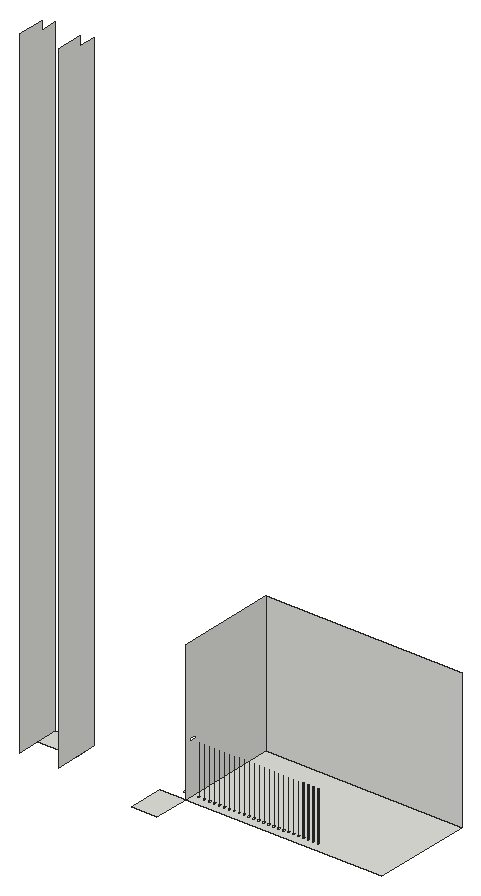
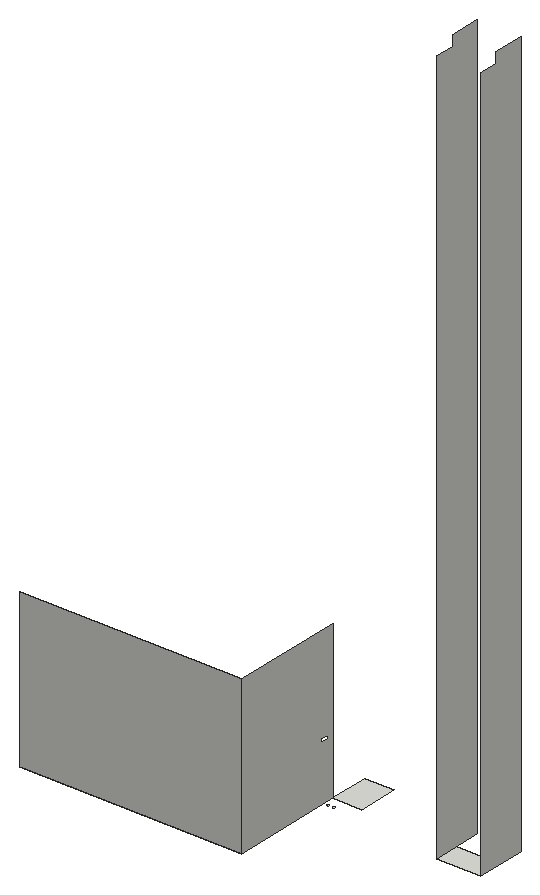
# SketchUp Ruby script. Lengths in inches.
U = 1.inch
M = Sketchup.active_model
def pt(a) = Geom::Point3d.new(a.map { |v| v * U })
def face(e, loops, mat)
  f = e.add_face(loops[0].map { |a| pt(a) })
  loops[1..].each { |l| e.add_face(l.map { |a| pt(a) }).erase! }
  f.material = f.back_material = mat if mat
  f
end
# faces: each face lists its corners as indices into pts; further lists are holes
def faces(e, pts, list, mat = nil) = list.each { |f| face(e, (f[0].is_a?(Array) ? f : [f]).map { |l| l.map { |i| pts[i] } }, mat) }
# xy, xz, yz: faces in a plane at the given z, y or x. An outline is a flat list of corners, or four numbers for a rectangle; further outlines are holes
def ring(l) = l.size == 4 ? [[l[0], l[1]], [l[2], l[1]], [l[2], l[3]], [l[0], l[3]]] : l.each_slice(2).to_a
def flat(e, list, mat, &to3) = list.each { |f| face(e, (f[0].is_a?(Array) ? f : [f]).map { |l| ring(l).map { |u, v| to3.(u, v) } }, mat) }
def xy(e, z, list, mat = nil) = flat(e, list, mat) { |x, y| [x, y, z] }
def xz(e, y, list, mat = nil) = flat(e, list, mat) { |x, z| [x, y, z] }
def yz(e, x, list, mat = nil) = flat(e, list, mat) { |y, z| [x, y, z] }
def lines(e, pts, list) = list.each { |a, b| e.add_line(pt(pts[a]), pt(pts[b])) }
# prism: a flat outline (further loops are holes) pulled along v
def prism(e, loops, v, mat = nil)
  f = face(e, loops, mat); d = Geom::Vector3d.new(v.map { |x| x * U })
  f.pushpull(f.normal.samedirection?(d) ? d.length : -d.length)
end
def box(e, o, s, mat = nil) = prism(e, [[o, [o[0] + s[0], o[1], o[2]], [o[0] + s[0], o[1] + s[1], o[2]], [o[0], o[1] + s[1], o[2]]]], [0, 0, s[2]], mat)
def at(x, y, z, deg = 0) = Geom::Transformation.translation(pt([x, y, z])) * Geom::Transformation.rotation(ORIGIN, Z_AXIS, deg.degrees)
def axes(o, x, y, z) = Geom::Transformation.new([*x, 0, *y, 0, *z, 0, *pt(o).to_a, 1])
def part(name) = M.definitions.add(name)
# library, detail: a bought-in or finely detailed component or shape, given as its bounding box
def library(name, o, s) = part(name).tap { |d| box(d.entities, o, s) }
def detail(e, o, s) = box(e.add_group.entities, o, s)
def put(e, d, t, mat = nil) = e.add_instance(d, t).tap { |i| i.material = mat if mat }
def group(e, t, mat = nil) = e.add_group.tap { |g| g.transformation = t; g.material = mat if mat }.entities
root = M.entities
xy(root,204.9375,[[259.3125,81.125,290.4375,124.5],[110.7,124.5,157.47,150.6875],[[290.4375,124.5,528.75,246],[520.27,135.31,520.48,135.34,520.67,135.42,520.84,135.55,520.97,135.72,521.05,135.91,521.08,136.12,521.05,136.33,520.97,136.53,520.84,136.7,520.67,136.83,520.48,136.91,520.27,136.93,520.06,136.91,519.86,136.83,519.69,136.7,519.5625,136.53,519.48,136.33,519.45,136.12,519.48,135.91,519.5625,135.72,519.69,135.55,519.86,135.42,520.06,135.34],[514.2,135.31,514.41,135.34,514.61,135.42,514.78,135.55,514.91,135.72,514.99,135.91,515.02,136.12,514.99,136.33,514.91,136.53,514.78,136.7,514.61,136.83,514.41,136.91,514.2,136.93,513.99,136.91,513.8,136.83,513.63,136.7,513.5,136.53,513.42,136.33,513.39,136.12,513.42,135.91,513.5,135.72,513.63,135.55,513.8,135.42,513.99,135.34],[508.14,135.31,508.35,135.34,508.55,135.42,508.72,135.55,508.85,135.72,508.93,135.91,508.95,136.12,508.93,136.33,508.85,136.53,508.72,136.7,508.55,136.83,508.35,136.91,508.14,136.93,507.93,136.91,507.74,136.83,507.57,136.7,507.4375,136.53,507.36,136.33,507.33,136.12,507.36,135.91,507.4375,135.72,507.57,135.55,507.74,135.42,507.93,135.34],[502.27,135.31,502.48,135.34,502.67,135.42,502.84,135.55,502.97,135.72,503.05,135.91,503.08,136.12,503.05,136.33,502.97,136.53,502.84,136.7,502.67,136.83,502.48,136.91,502.27,136.93,502.06,136.91,501.86,136.83,501.69,136.7,501.5625,136.53,501.48,136.33,501.45,136.12,501.48,135.91,501.5625,135.72,501.69,135.55,501.86,135.42,502.06,135.34],[496.27,135.31,496.48,135.34,496.67,135.42,496.84,135.55,496.97,135.72,497.05,135.91,497.08,136.12,497.05,136.33,496.97,136.53,496.84,136.7,496.67,136.83,496.48,136.91,496.27,136.93,496.06,136.91,495.86,136.83,495.69,136.7,495.5625,136.53,495.48,136.33,495.45,136.12,495.48,135.91,495.5625,135.72,495.69,135.55,495.86,135.42,496.06,135.34],[490.27,135.31,490.48,135.34,490.67,135.42,490.84,135.55,490.97,135.72,491.05,135.91,491.08,136.12,491.05,136.33,490.97,136.53,490.84,136.7,490.67,136.83,490.48,136.91,490.27,136.93,490.06,136.91,489.86,136.83,489.69,136.7,489.5625,136.53,489.48,136.33,489.45,136.12,489.48,135.91,489.5625,135.72,489.69,135.55,489.86,135.42,490.06,135.34],[484.2,135.31,484.41,135.34,484.61,135.42,484.78,135.55,484.91,135.72,484.99,135.91,485.02,136.12,484.99,136.33,484.91,136.53,484.78,136.7,484.61,136.83,484.41,136.91,484.2,136.93,483.99,136.91,483.8,136.83,483.63,136.7,483.5,136.53,483.42,136.33,483.39,136.12,483.42,135.91,483.5,135.72,483.63,135.55,483.8,135.42,483.99,135.34],[478.27,135.31,478.48,135.34,478.67,135.42,478.84,135.55,478.97,135.72,479.05,135.91,479.08,136.12,479.05,136.33,478.97,136.53,478.84,136.7,478.67,136.83,478.48,136.91,478.27,136.93,478.06,136.91,477.86,136.83,477.69,136.7,477.5625,136.53,477.48,136.33,477.45,136.12,477.48,135.91,477.5625,135.72,477.69,135.55,477.86,135.42,478.06,135.34],[472.27,135.31,472.48,135.34,472.67,135.42,472.84,135.55,472.97,135.72,473.05,135.91,473.08,136.12,473.05,136.33,472.97,136.53,472.84,136.7,472.67,136.83,472.48,136.91,472.27,136.93,472.06,136.91,471.86,136.83,471.69,136.7,471.5625,136.53,471.48,136.33,471.45,136.12,471.48,135.91,471.5625,135.72,471.69,135.55,471.86,135.42,472.06,135.34],[466.27,135.31,466.48,135.34,466.67,135.42,466.84,135.55,466.97,135.72,467.05,135.91,467.08,136.12,467.05,136.33,466.97,136.53,466.84,136.7,466.67,136.83,466.48,136.91,466.27,136.93,466.06,136.91,465.86,136.83,465.69,136.7,465.5625,136.53,465.48,136.33,465.45,136.12,465.48,135.91,465.5625,135.72,465.69,135.55,465.86,135.42,466.06,135.34],[460.33,135.31,460.54,135.34,460.74,135.42,460.9,135.55,461.03,135.72,461.11,135.91,461.14,136.12,461.11,136.33,461.03,136.53,460.9,136.7,460.74,136.83,460.54,136.91,460.33,136.93,460.12,136.91,459.92,136.83,459.75,136.7,459.625,136.53,459.54,136.33,459.52,136.12,459.54,135.91,459.625,135.72,459.75,135.55,459.92,135.42,460.12,135.34],[454.33,135.31,454.54,135.34,454.74,135.42,454.9,135.55,455.03,135.72,455.11,135.91,455.14,136.12,455.11,136.33,455.03,136.53,454.9,136.7,454.74,136.83,454.54,136.91,454.33,136.93,454.12,136.91,453.92,136.83,453.75,136.7,453.625,136.53,453.54,136.33,453.52,136.12,453.54,135.91,453.625,135.72,453.75,135.55,453.92,135.42,454.12,135.34],[448.33,135.31,448.54,135.34,448.74,135.42,448.9,135.55,449.03,135.72,449.11,135.91,449.14,136.12,449.11,136.33,449.03,136.53,448.9,136.7,448.74,136.83,448.54,136.91,448.33,136.93,448.12,136.91,447.92,136.83,447.75,136.7,447.625,136.53,447.54,136.33,447.52,136.12,447.54,135.91,447.625,135.72,447.75,135.55,447.92,135.42,448.12,135.34],[442.33,135.31,442.54,135.34,442.74,135.42,442.9,135.55,443.03,135.72,443.11,135.91,443.14,136.12,443.11,136.33,443.03,136.53,442.9,136.7,442.74,136.83,442.54,136.91,442.33,136.93,442.12,136.91,441.92,136.83,441.75,136.7,441.625,136.53,441.54,136.33,441.52,136.12,441.54,135.91,441.625,135.72,441.75,135.55,441.92,135.42,442.12,135.34],[436.33,135.31,436.54,135.34,436.74,135.42,436.9,135.55,437.03,135.72,437.11,135.91,437.14,136.12,437.11,136.33,437.03,136.53,436.9,136.7,436.74,136.83,436.54,136.91,436.33,136.93,436.12,136.91,435.92,136.83,435.75,136.7,435.625,136.53,435.54,136.33,435.52,136.12,435.54,135.91,435.625,135.72,435.75,135.55,435.92,135.42,436.12,135.34],[430.33,135.31,430.54,135.34,430.74,135.42,430.9,135.55,431.03,135.72,431.11,135.91,431.14,136.12,431.11,136.33,431.03,136.53,430.9,136.7,430.74,136.83,430.54,136.91,430.33,136.93,430.12,136.91,429.92,136.83,429.75,136.7,429.625,136.53,429.54,136.33,429.52,136.12,429.54,135.91,429.625,135.72,429.75,135.55,429.92,135.42,430.12,135.34],[424.33,135.31,424.54,135.34,424.74,135.42,424.9,135.55,425.03,135.72,425.11,135.91,425.14,136.12,425.11,136.33,425.03,136.53,424.9,136.7,424.74,136.83,424.54,136.91,424.33,136.93,424.12,136.91,423.92,136.83,423.75,136.7,423.625,136.53,423.54,136.33,423.52,136.12,423.54,135.91,423.625,135.72,423.75,135.55,423.92,135.42,424.12,135.34],[418.33,135.31,418.54,135.34,418.74,135.42,418.9,135.55,419.03,135.72,419.11,135.91,419.14,136.12,419.11,136.33,419.03,136.53,418.9,136.7,418.74,136.83,418.54,136.91,418.33,136.93,418.12,136.91,417.92,136.83,417.75,136.7,417.625,136.53,417.54,136.33,417.52,136.12,417.54,135.91,417.625,135.72,417.75,135.55,417.92,135.42,418.12,135.34],[412.33,135.31,412.54,135.34,412.74,135.42,412.9,135.55,413.03,135.72,413.11,135.91,413.14,136.12,413.11,136.33,413.03,136.53,412.9,136.7,412.74,136.83,412.54,136.91,412.33,136.93,412.12,136.91,411.92,136.83,411.75,136.7,411.625,136.53,411.54,136.33,411.52,136.12,411.54,135.91,411.625,135.72,411.75,135.55,411.92,135.42,412.12,135.34],[406.33,135.31,406.54,135.34,406.74,135.42,406.9,135.55,407.03,135.72,407.11,135.91,407.14,136.12,407.11,136.33,407.03,136.53,406.9,136.7,406.74,136.83,406.54,136.91,406.33,136.93,406.12,136.91,405.92,136.83,405.75,136.7,405.625,136.53,405.54,136.33,405.52,136.12,405.54,135.91,405.625,135.72,405.75,135.55,405.92,135.42,406.12,135.34],[400.33,135.31,400.54,135.34,400.74,135.42,400.9,135.55,401.03,135.72,401.11,135.91,401.14,136.12,401.11,136.33,401.03,136.53,400.9,136.7,400.74,136.83,400.54,136.91,400.33,136.93,400.12,136.91,399.92,136.83,399.75,136.7,399.625,136.53,399.54,136.33,399.52,136.12,399.54,135.91,399.625,135.72,399.75,135.55,399.92,135.42,400.12,135.34],[394.2,135.31,394.41,135.34,394.61,135.42,394.78,135.55,394.91,135.72,394.99,135.91,395.02,136.12,394.99,136.33,394.91,136.53,394.78,136.7,394.61,136.83,394.41,136.91,394.2,136.93,393.99,136.91,393.8,136.83,393.63,136.7,393.5,136.53,393.42,136.33,393.39,136.12,393.42,135.91,393.5,135.72,393.63,135.55,393.8,135.42,393.99,135.34],[388.08,135.31,388.29,135.34,388.49,135.42,388.65,135.55,388.78,135.72,388.86,135.91,388.89,136.12,388.86,136.33,388.78,136.53,388.65,136.7,388.49,136.83,388.29,136.91,388.08,136.93,387.87,136.91,387.67,136.83,387.5,136.7,387.375,136.53,387.29,136.33,387.27,136.12,387.29,135.91,387.375,135.72,387.5,135.55,387.67,135.42,387.87,135.34],[382.27,135.31,382.48,135.34,382.67,135.42,382.84,135.55,382.97,135.72,383.05,135.91,383.08,136.12,383.05,136.33,382.97,136.53,382.84,136.7,382.67,136.83,382.48,136.91,382.27,136.93,382.06,136.91,381.86,136.83,381.69,136.7,381.5625,136.53,381.48,136.33,381.45,136.12,381.48,135.91,381.5625,135.72,381.69,135.55,381.86,135.42,382.06,135.34],[376.27,135.31,376.48,135.34,376.67,135.42,376.84,135.55,376.97,135.72,377.05,135.91,377.08,136.12,377.05,136.33,376.97,136.53,376.84,136.7,376.67,136.83,376.48,136.91,376.27,136.93,376.06,136.91,375.86,136.83,375.69,136.7,375.5625,136.53,375.48,136.33,375.45,136.12,375.48,135.91,375.5625,135.72,375.69,135.55,375.86,135.42,376.06,135.34],[370.2,135.31,370.41,135.34,370.61,135.42,370.78,135.55,370.91,135.72,370.99,135.91,371.02,136.12,370.99,136.33,370.91,136.53,370.78,136.7,370.61,136.83,370.41,136.91,370.2,136.93,369.99,136.91,369.8,136.83,369.63,136.7,369.5,136.53,369.42,136.33,369.39,136.12,369.42,135.91,369.5,135.72,369.63,135.55,369.8,135.42,369.99,135.34],[364.27,135.31,364.48,135.34,364.67,135.42,364.84,135.55,364.97,135.72,365.05,135.91,365.08,136.12,365.05,136.33,364.97,136.53,364.84,136.7,364.67,136.83,364.48,136.91,364.27,136.93,364.06,136.91,363.86,136.83,363.69,136.7,363.5625,136.53,363.48,136.33,363.45,136.12,363.48,135.91,363.5625,135.72,363.69,135.55,363.86,135.42,364.06,135.34],[352.27,135.31,352.48,135.34,352.67,135.42,352.84,135.55,352.97,135.72,353.05,135.91,353.08,136.12,353.05,136.33,352.97,136.53,352.84,136.7,352.67,136.83,352.48,136.91,352.27,136.93,352.06,136.91,351.86,136.83,351.69,136.7,351.5625,136.53,351.48,136.33,351.45,136.12,351.48,135.91,351.5625,135.72,351.69,135.55,351.86,135.42,352.06,135.34],[346.27,135.31,346.48,135.34,346.67,135.42,346.84,135.55,346.97,135.72,347.05,135.91,347.08,136.12,347.05,136.33,346.97,136.53,346.84,136.7,346.67,136.83,346.48,136.91,346.27,136.93,346.06,136.91,345.86,136.83,345.69,136.7,345.5625,136.53,345.48,136.33,345.45,136.12,345.48,135.91,345.5625,135.72,345.69,135.55,345.86,135.42,346.06,135.34],[340.27,135.31,340.48,135.34,340.67,135.42,340.84,135.55,340.97,135.72,341.05,135.91,341.08,136.12,341.05,136.33,340.97,136.53,340.84,136.7,340.67,136.83,340.48,136.91,340.27,136.93,340.06,136.91,339.86,136.83,339.69,136.7,339.5625,136.53,339.48,136.33,339.45,136.12,339.48,135.91,339.5625,135.72,339.69,135.55,339.86,135.42,340.06,135.34],[358.27,135.31,358.48,135.34,358.67,135.42,358.84,135.55,358.97,135.72,359.05,135.91,359.08,136.12,359.05,136.33,358.97,136.53,358.84,136.7,358.67,136.83,358.48,136.91,358.27,136.93,358.06,136.91,357.86,136.83,357.69,136.7,357.5625,136.53,357.48,136.33,357.45,136.12,357.48,135.91,357.5625,135.72,357.69,135.55,357.86,135.42,358.06,135.34],[334.27,135.31,334.48,135.34,334.67,135.42,334.84,135.55,334.97,135.72,335.05,135.91,335.08,136.12,335.05,136.33,334.97,136.53,334.84,136.7,334.67,136.83,334.48,136.91,334.27,136.93,334.06,136.91,333.86,136.83,333.69,136.7,333.5625,136.53,333.48,136.33,333.45,136.12,333.48,135.91,333.5625,135.72,333.69,135.55,333.86,135.42,334.06,135.34],[328.27,135.31,328.48,135.34,328.67,135.42,328.84,135.55,328.97,135.72,329.05,135.91,329.08,136.12,329.05,136.33,328.97,136.53,328.84,136.7,328.67,136.83,328.48,136.91,328.27,136.93,328.06,136.91,327.86,136.83,327.69,136.7,327.5625,136.53,327.48,136.33,327.45,136.12,327.48,135.91,327.5625,135.72,327.69,135.55,327.86,135.42,328.06,135.34],[322.27,135.31,322.48,135.34,322.67,135.42,322.84,135.55,322.97,135.72,323.05,135.91,323.08,136.12,323.05,136.33,322.97,136.53,322.84,136.7,322.67,136.83,322.48,136.91,322.27,136.93,322.06,136.91,321.86,136.83,321.69,136.7,321.5625,136.53,321.48,136.33,321.45,136.12,321.48,135.91,321.5625,135.72,321.69,135.55,321.86,135.42,322.06,135.34],[316.27,135.31,316.48,135.34,316.67,135.42,316.84,135.55,316.97,135.72,317.05,135.91,317.08,136.12,317.05,136.33,316.97,136.53,316.84,136.7,316.67,136.83,316.48,136.91,316.27,136.93,316.06,136.91,315.86,136.83,315.69,136.7,315.5625,136.53,315.48,136.33,315.45,136.12,315.48,135.91,315.5625,135.72,315.69,135.55,315.86,135.42,316.06,135.34],[310.27,135.31,310.48,135.34,310.67,135.42,310.84,135.55,310.97,135.72,311.05,135.91,311.08,136.12,311.05,136.33,310.97,136.53,310.84,136.7,310.67,136.83,310.48,136.91,310.27,136.93,310.06,136.91,309.86,136.83,309.69,136.7,309.5625,136.53,309.48,136.33,309.45,136.12,309.48,135.91,309.5625,135.72,309.69,135.55,309.86,135.42,310.06,135.34],[303.89,135.31,304.1,135.34,304.3,135.42,304.47,135.55,304.6,135.72,304.68,135.91,304.7,136.12,304.68,136.33,304.6,136.53,304.47,136.7,304.3,136.83,304.1,136.91,303.89,136.93,303.68,136.91,303.49,136.83,303.32,136.7,303.1875,136.53,303.11,136.33,303.08,136.12,303.11,135.91,303.1875,135.72,303.32,135.55,303.49,135.42,303.68,135.34],[297.27,135.31,297.48,135.34,297.67,135.42,297.84,135.55,297.97,135.72,298.05,135.91,298.08,136.12,298.05,136.33,297.97,136.53,297.84,136.7,297.67,136.83,297.48,136.91,297.27,136.93,297.06,136.91,296.86,136.83,296.69,136.7,296.5625,136.53,296.48,136.33,296.45,136.12,296.48,135.91,296.5625,135.72,296.69,135.55,296.86,135.42,297.06,135.34]],[280.27,135.31,280.06,135.34,279.86,135.42,279.69,135.55,279.5625,135.72,279.48,135.91,279.45,136.12,279.48,136.33,279.5625,136.53,279.69,136.7,279.86,136.83,280.06,136.91,280.27,136.93,280.48,136.91,280.67,136.83,280.84,136.7,280.97,136.53,281.05,136.33,281.08,136.12,281.05,135.91,280.97,135.72,280.84,135.55,280.67,135.42,280.48,135.34],[286.27,135.31,286.06,135.34,285.86,135.42,285.69,135.55,285.5625,135.72,285.48,135.91,285.45,136.12,285.48,136.33,285.5625,136.53,285.69,136.7,285.86,136.83,286.06,136.91,286.27,136.93,286.48,136.91,286.67,136.83,286.84,136.7,286.97,136.53,287.05,136.33,287.08,136.12,287.05,135.91,286.97,135.72,286.84,135.55,286.67,135.42,286.48,135.34],
  [297.27,135.31,297.06,135.34,296.86,135.42,296.69,135.55,296.5625,135.72,296.48,135.91,296.45,136.12,296.48,136.33,296.5625,136.53,296.69,136.7,296.86,136.83,297.06,136.91,297.27,136.93,297.48,136.91,297.67,136.83,297.84,136.7,297.97,136.53,298.05,136.33,298.08,136.12,298.05,135.91,297.97,135.72,297.84,135.55,297.67,135.42,297.48,135.34],[303.89,135.31,303.68,135.34,303.49,135.42,303.32,135.55,303.1875,135.72,303.11,135.91,303.08,136.12,303.11,136.33,303.1875,136.53,303.32,136.7,303.49,136.83,303.68,136.91,303.89,136.93,304.1,136.91,304.3,136.83,304.47,136.7,304.6,136.53,304.68,136.33,304.7,136.12,304.68,135.91,304.6,135.72,304.47,135.55,304.3,135.42,304.1,135.34],[310.27,135.31,310.06,135.34,309.86,135.42,309.69,135.55,309.5625,135.72,309.48,135.91,309.45,136.12,309.48,136.33,309.5625,136.53,309.69,136.7,309.86,136.83,310.06,136.91,310.27,136.93,310.48,136.91,310.67,136.83,310.84,136.7,310.97,136.53,311.05,136.33,311.08,136.12,311.05,135.91,310.97,135.72,310.84,135.55,310.67,135.42,310.48,135.34],[316.27,135.31,316.06,135.34,315.86,135.42,315.69,135.55,315.5625,135.72,315.48,135.91,315.45,136.12,315.48,136.33,315.5625,136.53,315.69,136.7,315.86,136.83,316.06,136.91,316.27,136.93,316.48,136.91,316.67,136.83,316.84,136.7,316.97,136.53,317.05,136.33,317.08,136.12,317.05,135.91,316.97,135.72,316.84,135.55,316.67,135.42,316.48,135.34],[322.27,135.31,322.06,135.34,321.86,135.42,321.69,135.55,321.5625,135.72,321.48,135.91,321.45,136.12,321.48,136.33,321.5625,136.53,321.69,136.7,321.86,136.83,322.06,136.91,322.27,136.93,322.48,136.91,322.67,136.83,322.84,136.7,322.97,136.53,323.05,136.33,323.08,136.12,323.05,135.91,322.97,135.72,322.84,135.55,322.67,135.42,322.48,135.34],
  [328.27,135.31,328.06,135.34,327.86,135.42,327.69,135.55,327.5625,135.72,327.48,135.91,327.45,136.12,327.48,136.33,327.5625,136.53,327.69,136.7,327.86,136.83,328.06,136.91,328.27,136.93,328.48,136.91,328.67,136.83,328.84,136.7,328.97,136.53,329.05,136.33,329.08,136.12,329.05,135.91,328.97,135.72,328.84,135.55,328.67,135.42,328.48,135.34],[334.27,135.31,334.06,135.34,333.86,135.42,333.69,135.55,333.5625,135.72,333.48,135.91,333.45,136.12,333.48,136.33,333.5625,136.53,333.69,136.7,333.86,136.83,334.06,136.91,334.27,136.93,334.48,136.91,334.67,136.83,334.84,136.7,334.97,136.53,335.05,136.33,335.08,136.12,335.05,135.91,334.97,135.72,334.84,135.55,334.67,135.42,334.48,135.34],[340.27,135.31,340.06,135.34,339.86,135.42,339.69,135.55,339.5625,135.72,339.48,135.91,339.45,136.12,339.48,136.33,339.5625,136.53,339.69,136.7,339.86,136.83,340.06,136.91,340.27,136.93,340.48,136.91,340.67,136.83,340.84,136.7,340.97,136.53,341.05,136.33,341.08,136.12,341.05,135.91,340.97,135.72,340.84,135.55,340.67,135.42,340.48,135.34],[346.27,135.31,346.06,135.34,345.86,135.42,345.69,135.55,345.5625,135.72,345.48,135.91,345.45,136.12,345.48,136.33,345.5625,136.53,345.69,136.7,345.86,136.83,346.06,136.91,346.27,136.93,346.48,136.91,346.67,136.83,346.84,136.7,346.97,136.53,347.05,136.33,347.08,136.12,347.05,135.91,346.97,135.72,346.84,135.55,346.67,135.42,346.48,135.34],[352.27,135.31,352.06,135.34,351.86,135.42,351.69,135.55,351.5625,135.72,351.48,135.91,351.45,136.12,351.48,136.33,351.5625,136.53,351.69,136.7,351.86,136.83,352.06,136.91,352.27,136.93,352.48,136.91,352.67,136.83,352.84,136.7,352.97,136.53,353.05,136.33,353.08,136.12,353.05,135.91,352.97,135.72,352.84,135.55,352.67,135.42,352.48,135.34],
  [358.27,135.31,358.06,135.34,357.86,135.42,357.69,135.55,357.5625,135.72,357.48,135.91,357.45,136.12,357.48,136.33,357.5625,136.53,357.69,136.7,357.86,136.83,358.06,136.91,358.27,136.93,358.48,136.91,358.67,136.83,358.84,136.7,358.97,136.53,359.05,136.33,359.08,136.12,359.05,135.91,358.97,135.72,358.84,135.55,358.67,135.42,358.48,135.34],[364.27,135.31,364.06,135.34,363.86,135.42,363.69,135.55,363.5625,135.72,363.48,135.91,363.45,136.12,363.48,136.33,363.5625,136.53,363.69,136.7,363.86,136.83,364.06,136.91,364.27,136.93,364.48,136.91,364.67,136.83,364.84,136.7,364.97,136.53,365.05,136.33,365.08,136.12,365.05,135.91,364.97,135.72,364.84,135.55,364.67,135.42,364.48,135.34],[370.2,135.31,369.99,135.34,369.8,135.42,369.63,135.55,369.5,135.72,369.42,135.91,369.39,136.12,369.42,136.33,369.5,136.53,369.63,136.7,369.8,136.83,369.99,136.91,370.2,136.93,370.41,136.91,370.61,136.83,370.78,136.7,370.91,136.53,370.99,136.33,371.02,136.12,370.99,135.91,370.91,135.72,370.78,135.55,370.61,135.42,370.41,135.34],[376.27,135.31,376.06,135.34,375.86,135.42,375.69,135.55,375.5625,135.72,375.48,135.91,375.45,136.12,375.48,136.33,375.5625,136.53,375.69,136.7,375.86,136.83,376.06,136.91,376.27,136.93,376.48,136.91,376.67,136.83,376.84,136.7,376.97,136.53,377.05,136.33,377.08,136.12,377.05,135.91,376.97,135.72,376.84,135.55,376.67,135.42,376.48,135.34],[382.27,135.31,382.06,135.34,381.86,135.42,381.69,135.55,381.5625,135.72,381.48,135.91,381.45,136.12,381.48,136.33,381.5625,136.53,381.69,136.7,381.86,136.83,382.06,136.91,382.27,136.93,382.48,136.91,382.67,136.83,382.84,136.7,382.97,136.53,383.05,136.33,383.08,136.12,383.05,135.91,382.97,135.72,382.84,135.55,382.67,135.42,382.48,135.34],
  [388.08,135.31,387.87,135.34,387.67,135.42,387.5,135.55,387.375,135.72,387.29,135.91,387.27,136.12,387.29,136.33,387.375,136.53,387.5,136.7,387.67,136.83,387.87,136.91,388.08,136.93,388.29,136.91,388.49,136.83,388.65,136.7,388.78,136.53,388.86,136.33,388.89,136.12,388.86,135.91,388.78,135.72,388.65,135.55,388.49,135.42,388.29,135.34],[394.2,135.31,393.99,135.34,393.8,135.42,393.63,135.55,393.5,135.72,393.42,135.91,393.39,136.12,393.42,136.33,393.5,136.53,393.63,136.7,393.8,136.83,393.99,136.91,394.2,136.93,394.41,136.91,394.61,136.83,394.78,136.7,394.91,136.53,394.99,136.33,395.02,136.12,394.99,135.91,394.91,135.72,394.78,135.55,394.61,135.42,394.41,135.34],[400.33,135.31,400.12,135.34,399.92,135.42,399.75,135.55,399.625,135.72,399.54,135.91,399.52,136.12,399.54,136.33,399.625,136.53,399.75,136.7,399.92,136.83,400.12,136.91,400.33,136.93,400.54,136.91,400.74,136.83,400.9,136.7,401.03,136.53,401.11,136.33,401.14,136.12,401.11,135.91,401.03,135.72,400.9,135.55,400.74,135.42,400.54,135.34],[406.33,135.31,406.12,135.34,405.92,135.42,405.75,135.55,405.625,135.72,405.54,135.91,405.52,136.12,405.54,136.33,405.625,136.53,405.75,136.7,405.92,136.83,406.12,136.91,406.33,136.93,406.54,136.91,406.74,136.83,406.9,136.7,407.03,136.53,407.11,136.33,407.14,136.12,407.11,135.91,407.03,135.72,406.9,135.55,406.74,135.42,406.54,135.34],[412.33,135.31,412.12,135.34,411.92,135.42,411.75,135.55,411.625,135.72,411.54,135.91,411.52,136.12,411.54,136.33,411.625,136.53,411.75,136.7,411.92,136.83,412.12,136.91,412.33,136.93,412.54,136.91,412.74,136.83,412.9,136.7,413.03,136.53,413.11,136.33,413.14,136.12,413.11,135.91,413.03,135.72,412.9,135.55,412.74,135.42,412.54,135.34],
  [418.33,135.31,418.12,135.34,417.92,135.42,417.75,135.55,417.625,135.72,417.54,135.91,417.52,136.12,417.54,136.33,417.625,136.53,417.75,136.7,417.92,136.83,418.12,136.91,418.33,136.93,418.54,136.91,418.74,136.83,418.9,136.7,419.03,136.53,419.11,136.33,419.14,136.12,419.11,135.91,419.03,135.72,418.9,135.55,418.74,135.42,418.54,135.34],[424.33,135.31,424.12,135.34,423.92,135.42,423.75,135.55,423.625,135.72,423.54,135.91,423.52,136.12,423.54,136.33,423.625,136.53,423.75,136.7,423.92,136.83,424.12,136.91,424.33,136.93,424.54,136.91,424.74,136.83,424.9,136.7,425.03,136.53,425.11,136.33,425.14,136.12,425.11,135.91,425.03,135.72,424.9,135.55,424.74,135.42,424.54,135.34],[430.33,135.31,430.12,135.34,429.92,135.42,429.75,135.55,429.625,135.72,429.54,135.91,429.52,136.12,429.54,136.33,429.625,136.53,429.75,136.7,429.92,136.83,430.12,136.91,430.33,136.93,430.54,136.91,430.74,136.83,430.9,136.7,431.03,136.53,431.11,136.33,431.14,136.12,431.11,135.91,431.03,135.72,430.9,135.55,430.74,135.42,430.54,135.34],[436.33,135.31,436.12,135.34,435.92,135.42,435.75,135.55,435.625,135.72,435.54,135.91,435.52,136.12,435.54,136.33,435.625,136.53,435.75,136.7,435.92,136.83,436.12,136.91,436.33,136.93,436.54,136.91,436.74,136.83,436.9,136.7,437.03,136.53,437.11,136.33,437.14,136.12,437.11,135.91,437.03,135.72,436.9,135.55,436.74,135.42,436.54,135.34],[442.33,135.31,442.12,135.34,441.92,135.42,441.75,135.55,441.625,135.72,441.54,135.91,441.52,136.12,441.54,136.33,441.625,136.53,441.75,136.7,441.92,136.83,442.12,136.91,442.33,136.93,442.54,136.91,442.74,136.83,442.9,136.7,443.03,136.53,443.11,136.33,443.14,136.12,443.11,135.91,443.03,135.72,442.9,135.55,442.74,135.42,442.54,135.34]])
xz(root,246,[[290.4375,204.9375,528.75,372.9375]])
yz(root,110.7,[[97.25,204.9375,150.6875,204.9375,150.6875,976.6875,130.3125,976.6875,130.3125,987.75,97.25,987.75]])
yz(root,157.47,[[97.25,204.9375,97.25,239.9375,98,239.9375,98,240.4375,97.25,240.4375,97.25,453.4375,98.375,453.4375,98.375,453.9375,97.25,453.9375,97.25,513.6875,98.375,513.6875,98.375,514.1875,97.25,514.1875,97.25,667,98,667,98,667.5,97.25,667.5,97.25,728.25,98,728.25,98,728.75,97.25,728.75,97.25,879.5,98,879.5,98,880,97.25,880,97.25,943.1875,98,943.1875,98,943.6875,97.25,943.6875,97.25,987.75,130.3125,987.75,130.3125,976.6875,150.6875,976.6875,150.6875,204.9375]])
yz(root,290.4375,[[[124.5,204.9375,246,372.9375],[130.75,264.83,140.05,269.02]]])
p = [[429.92,135.42,204.9375],[430.12,135.34,204.9375],[430.12,135.34,264.83],[429.92,135.42,264.83],[430.33,135.31,204.9375],[430.33,135.31,264.83],
  [430.54,135.34,204.9375],[430.54,135.34,264.83],[430.74,135.42,204.9375],[430.74,135.42,264.83],[435.92,135.42,204.9375],[436.12,135.34,204.9375],
  [436.12,135.34,264.83],[435.92,135.42,264.83],[436.33,135.31,204.9375],[436.33,135.31,264.83],[436.54,135.34,204.9375],[436.54,135.34,264.83],
  [436.74,135.42,204.9375],[436.74,135.42,264.83],[441.92,135.42,204.9375],[442.12,135.34,204.9375],[442.12,135.34,264.83],[441.92,135.42,264.83],
  [442.33,135.31,204.9375],[442.33,135.31,264.83],[442.54,135.34,204.9375],[442.54,135.34,264.83],[442.74,135.42,204.9375],[442.74,135.42,264.83],
  [429.75,135.55,204.9375],[429.75,135.55,264.83],[430.9,135.55,204.9375],[430.9,135.55,264.83],[435.75,135.55,204.9375],[435.75,135.55,264.83],
  [436.9,135.55,204.9375],[436.9,135.55,264.83],[441.75,135.55,204.9375],[441.75,135.55,264.83],[442.9,135.55,204.9375],[442.9,135.55,264.83],
  [429.625,135.72,204.9375],[429.625,135.72,264.83],[431.03,135.72,204.9375],[431.03,135.72,264.83],[435.625,135.72,204.9375],[435.625,135.72,264.83],
  [437.03,135.72,204.9375],[437.03,135.72,264.83],[441.625,135.72,204.9375],[441.625,135.72,264.83],[443.03,135.72,204.9375],[443.03,135.72,264.83],
  [429.54,135.91,204.9375],[429.54,135.91,264.83],[431.11,135.91,204.9375],[431.11,135.91,264.83],[435.54,135.91,204.9375],[435.54,135.91,264.83],
  [437.11,135.91,204.9375],[437.11,135.91,264.83],[441.54,135.91,204.9375],[441.54,135.91,264.83],[423.52,136.12,204.9375],[423.54,135.91,204.9375],
  [423.54,135.91,264.83],[423.52,136.12,264.83],[429.52,136.12,204.9375],[429.52,136.12,264.83],[431.14,136.12,204.9375],[431.14,136.12,264.83],
  [435.52,136.12,204.9375],[435.52,136.12,264.83],[437.14,136.12,204.9375],[437.14,136.12,264.83],[441.52,136.12,204.9375],[441.52,136.12,264.83],
  [423.54,136.33,204.9375],[423.54,136.33,264.83],[429.54,136.33,204.9375],[429.54,136.33,264.83],[431.11,136.33,204.9375],[431.11,136.33,264.83],
  [435.54,136.33,204.9375],[435.54,136.33,264.83],[437.11,136.33,204.9375],[437.11,136.33,264.83],[441.54,136.33,204.9375],[441.54,136.33,264.83],
  [423.625,136.53,204.9375],[423.625,136.53,264.83],[429.625,136.53,204.9375],[429.625,136.53,264.83],[431.03,136.53,204.9375],[431.03,136.53,264.83],
  [435.625,136.53,204.9375],[435.625,136.53,264.83],[437.03,136.53,204.9375],[437.03,136.53,264.83],[441.625,136.53,204.9375],[441.625,136.53,264.83],
  [443.11,136.33,204.9375],[443.03,136.53,204.9375],[443.03,136.53,264.83],[443.11,136.33,264.83],[423.75,136.7,204.9375],[423.75,136.7,264.83],
  [429.75,136.7,204.9375],[429.75,136.7,264.83],[430.9,136.7,204.9375],[430.9,136.7,264.83],[435.75,136.7,204.9375],[435.75,136.7,264.83],
  [436.9,136.7,204.9375],[436.9,136.7,264.83],[441.75,136.7,204.9375],[441.75,136.7,264.83],[442.9,136.7,204.9375],[442.9,136.7,264.83],
  [423.92,136.83,204.9375],[423.92,136.83,264.83],[429.92,136.83,204.9375],[429.92,136.83,264.83],[430.74,136.83,204.9375],[430.74,136.83,264.83],
  [435.92,136.83,204.9375],[435.92,136.83,264.83],[436.74,136.83,204.9375],[436.74,136.83,264.83],[441.92,136.83,204.9375],[441.92,136.83,264.83],
  [442.74,136.83,204.9375],[442.74,136.83,264.83],[424.12,136.91,204.9375],[424.12,136.91,264.83],[430.12,136.91,204.9375],[430.12,136.91,264.83],
  [430.54,136.91,204.9375],[430.54,136.91,264.83],[436.12,136.91,204.9375],[436.12,136.91,264.83],[436.54,136.91,204.9375],[436.54,136.91,264.83],
  [442.12,136.91,204.9375],[442.12,136.91,264.83],[442.54,136.91,204.9375],[442.54,136.91,264.83],[424.33,136.93,204.9375],[424.33,136.93,264.83],
  [424.54,136.91,204.9375],[424.54,136.91,264.83],[430.33,136.93,204.9375],[430.33,136.93,264.83],[436.33,136.93,204.9375],[436.33,136.93,264.83],
  [442.33,136.93,204.9375],[442.33,136.93,264.83],[442.27,136.12,264.83],[442.27,136.12,204.9375],[436.27,136.12,264.83],[436.27,136.12,204.9375],
  [430.27,136.12,264.83],[430.27,136.12,204.9375],[424.27,136.12,264.83],[424.27,136.12,204.9375],[418.27,136.12,264.83],[418.27,136.12,204.9375],
  [412.27,136.12,264.83],[412.27,136.12,204.9375],[406.27,136.12,264.83],[406.27,136.12,204.9375],[400.27,136.12,264.83],[400.27,136.12,204.9375],
  [394.27,136.12,264.83],[394.27,136.12,204.9375],[388.27,136.12,264.83],[388.27,136.12,204.9375],[382.27,136.12,264.83],[382.27,136.12,204.9375],
  [376.27,136.12,264.83],[376.27,136.12,204.9375],[370.27,136.12,264.83],[370.27,136.12,204.9375],[364.27,136.12,264.83],[364.27,136.12,204.9375],
  [358.27,136.12,264.83],[358.27,136.12,204.9375],[352.27,136.12,264.83],[352.27,136.12,204.9375],[346.27,136.12,264.83],[346.27,136.12,204.9375],
  [340.27,136.12,264.83],[340.27,136.12,204.9375],[334.27,136.12,264.83],[334.27,136.12,204.9375],[328.27,136.12,264.83],[328.27,136.12,204.9375],
  [322.27,136.12,264.83],[322.27,136.12,204.9375],[316.27,136.12,264.83],[316.27,136.12,204.9375],[310.27,136.12,264.83],[310.27,136.12,204.9375],
  [303.77,136.12,264.83],[303.77,136.12,204.9375],[297.27,136.12,264.83],[297.27,136.12,204.9375]]
faces(root,p,[[0,1,2,3],[1,4,5,2],[4,6,7,5],[6,8,9,7],[10,11,12,13],[11,14,15,12],[14,16,17,15],[16,18,19,17],
  [20,21,22,23],[21,24,25,22],[24,26,27,25],[26,28,29,27],[30,0,3,31],[8,32,33,9],[34,10,13,35],[18,36,37,19],
  [38,20,23,39],[28,40,41,29],[42,30,31,43],[32,44,45,33],[46,34,35,47],[36,48,49,37],[50,38,39,51],[40,52,53,41],
  [54,42,43,55],[44,56,57,45],[58,46,47,59],[48,60,61,49],[62,50,51,63],[64,65,66,67],[68,54,55,69],[56,70,71,57],
  [72,58,59,73],[60,74,75,61],[76,62,63,77],[78,64,67,79],[80,68,69,81],[70,82,83,71],[84,72,73,85],[74,86,87,75],
  [88,76,77,89],[90,78,79,91],[92,80,81,93],[82,94,95,83],[96,84,85,97],[86,98,99,87],[100,88,89,101],[102,103,104,105],
  [106,90,91,107],[108,92,93,109],[94,110,111,95],[112,96,97,113],[98,114,115,99],[116,100,101,117],[103,118,119,104],[120,106,107,121],
  [122,108,109,123],[110,124,125,111],[126,112,113,127],[114,128,129,115],[130,116,117,131],[118,132,133,119],[134,120,121,135],[136,122,123,137],
  [124,138,139,125],[140,126,127,141],[128,142,143,129],[144,130,131,145],[132,146,147,133],[148,134,135,149],[150,148,149,151],[152,136,137,153],
  [138,152,153,139],[154,140,141,155],[142,154,155,143],[156,144,145,157],[146,156,157,147]])
lines(root,p,[[158,159],[160,161],[162,163],[164,165],[166,167],[168,169],[170,171],[172,173],[174,175],[176,177],[178,179],[180,181],
  [182,183],[184,185],[186,187],[188,189],[190,191],[192,193],[194,195],[196,197],[198,199],[200,201],[202,203],[204,205],
  [206,207]])
